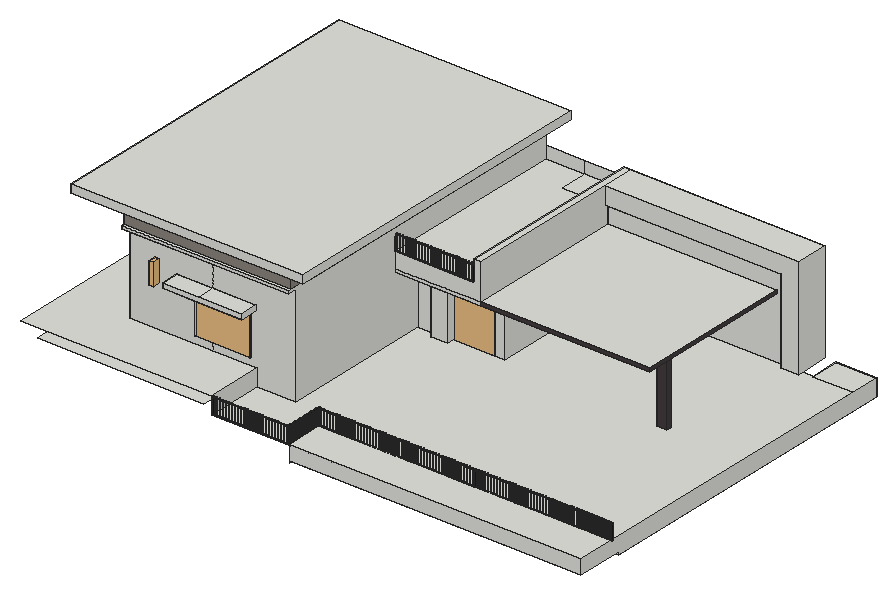
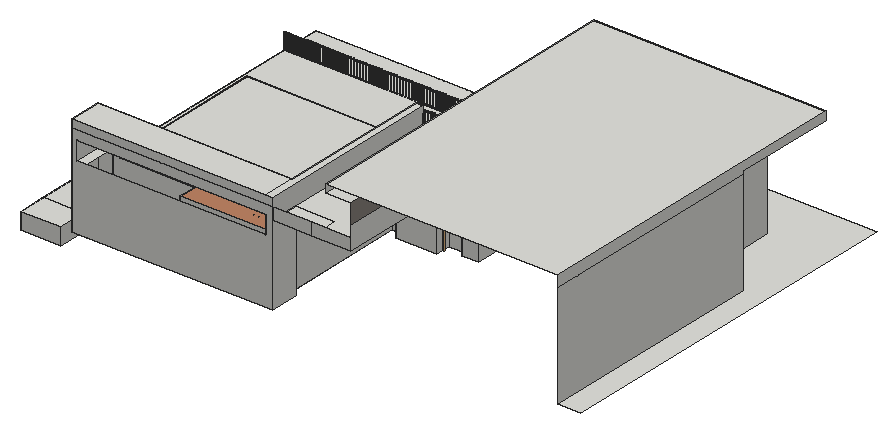
# SketchUp Ruby script. Lengths in inches.
U = 1.inch
M = Sketchup.active_model
def pt(a) = Geom::Point3d.new(a.map { |v| v * U })
def face(e, loops, mat)
  f = e.add_face(loops[0].map { |a| pt(a) })
  loops[1..].each { |l| e.add_face(l.map { |a| pt(a) }).erase! }
  f.material = f.back_material = mat if mat
  f
end
# faces: each face lists its corners as indices into pts; further lists are holes
def faces(e, pts, list, mat = nil) = list.each { |f| face(e, (f[0].is_a?(Array) ? f : [f]).map { |l| l.map { |i| pts[i] } }, mat) }
# xy, xz, yz: faces in a plane at the given z, y or x. An outline is a flat list of corners, or four numbers for a rectangle; further outlines are holes
def ring(l) = l.size == 4 ? [[l[0], l[1]], [l[2], l[1]], [l[2], l[3]], [l[0], l[3]]] : l.each_slice(2).to_a
def flat(e, list, mat, &to3) = list.each { |f| face(e, (f[0].is_a?(Array) ? f : [f]).map { |l| ring(l).map { |u, v| to3.(u, v) } }, mat) }
def xy(e, z, list, mat = nil) = flat(e, list, mat) { |x, y| [x, y, z] }
def xz(e, y, list, mat = nil) = flat(e, list, mat) { |x, z| [x, y, z] }
def yz(e, x, list, mat = nil) = flat(e, list, mat) { |y, z| [x, y, z] }
def lines(e, pts, list) = list.each { |a, b| e.add_line(pt(pts[a]), pt(pts[b])) }
# prism: a flat outline (further loops are holes) pulled along v
def prism(e, loops, v, mat = nil)
  f = face(e, loops, mat); d = Geom::Vector3d.new(v.map { |x| x * U })
  f.pushpull(f.normal.samedirection?(d) ? d.length : -d.length)
end
def box(e, o, s, mat = nil) = prism(e, [[o, [o[0] + s[0], o[1], o[2]], [o[0] + s[0], o[1] + s[1], o[2]], [o[0], o[1] + s[1], o[2]]]], [0, 0, s[2]], mat)
def at(x, y, z, deg = 0) = Geom::Transformation.translation(pt([x, y, z])) * Geom::Transformation.rotation(ORIGIN, Z_AXIS, deg.degrees)
def axes(o, x, y, z) = Geom::Transformation.new([*x, 0, *y, 0, *z, 0, *pt(o).to_a, 1])
def part(name) = M.definitions.add(name)
# library, detail: a bought-in or finely detailed component or shape, given as its bounding box
def library(name, o, s) = part(name).tap { |d| box(d.entities, o, s) }
def detail(e, o, s) = box(e.add_group.entities, o, s)
def put(e, d, t, mat = nil) = e.add_instance(d, t).tap { |i| i.material = mat if mat }
def group(e, t, mat = nil) = e.add_group.tap { |g| g.transformation = t; g.material = mat if mat }.entities
root = M.entities
M.materials.add("[Asphalt New]").color = [67, 60, 62]
M.materials.add("[Color M08]").color = [30, 30, 30]
M.materials.add("[Concrete Scored Jointless]").color = [140, 133, 127]
M.materials.add("[Modern Siding]").color = [191, 132, 100]
c1 = part("Group\#428")
prism(c1.entities,[[[0,1.97,0],[0,1.97,1.18],[0,0,1.18],[0,0,0]],[[0,1.92,1.13],[0,1.92,0.05],[0,0.05,0.05],[0,0.05,1.13]]],[98.43,0,0])
c2 = part("Group\#430")
xy(c2.entities,0,[[0.3,0,0.22,0.01,0.15,0.04,0.09,0.09,0.04,0.15,0.01,0.22,0,0.3,0.3,0.3],[0.3,0,0.3,0.3,0.59,0.3,0.58,0.22,0.55,0.15,0.5,0.09,0.44,0.04,0.37,0.01],[0,0.3,0.01,0.37,0.04,0.44,0.09,0.5,0.15,0.55,0.22,0.58,0.3,0.59,0.3,0.3],[0.3,0.3,0.3,0.59,0.37,0.58,0.44,0.55,0.5,0.5,0.55,0.44,0.58,0.37,0.59,0.3]])
xy(c2.entities,39.37,[[0.3,0,0.37,0.01,0.44,0.04,0.5,0.09,0.55,0.15,0.58,0.22,0.59,0.3,0.58,0.37,0.55,0.44,0.5,0.5,0.44,0.55,0.37,0.58,0.3,0.59,0.22,0.58,0.15,0.55,0.09,0.5,0.04,0.44,0.01,0.37,0,0.3,0.01,0.22,0.04,0.15,0.09,0.09,0.15,0.04,0.22,0.01]])
p = [[0.09,0.09,0],[0.15,0.04,0],[0.15,0.04,39.37],[0.09,0.09,39.37],[0.22,0.01,0],[0.22,0.01,39.37],
  [0.3,0,0],[0.3,0,39.37],[0.37,0.01,0],[0.37,0.01,39.37],[0.44,0.04,0],[0.44,0.04,39.37],
  [0.5,0.09,0],[0.5,0.09,39.37],[0.01,0.22,0],[0.04,0.15,0],[0.04,0.15,39.37],[0.01,0.22,39.37],
  [0.55,0.15,0],[0.55,0.15,39.37],[0.58,0.22,0],[0.58,0.22,39.37],[0,0.3,0],[0,0.3,39.37],
  [0.59,0.3,0],[0.59,0.3,39.37],[0.01,0.37,0],[0.01,0.37,39.37],[0.58,0.37,0],[0.58,0.37,39.37],
  [0.09,0.5,0],[0.04,0.44,0],[0.04,0.44,39.37],[0.09,0.5,39.37],[0.55,0.44,0],[0.5,0.5,0],
  [0.5,0.5,39.37],[0.55,0.44,39.37],[0.15,0.55,0],[0.15,0.55,39.37],[0.44,0.55,0],[0.44,0.55,39.37],
  [0.22,0.58,0],[0.22,0.58,39.37],[0.3,0.59,0],[0.3,0.59,39.37],[0.37,0.58,0],[0.37,0.58,39.37]]
faces(c2.entities,p,[[0,1,2,3],[1,4,5,2],[4,6,7,5],[6,8,9,7],[8,10,11,9],[10,12,13,11],[14,15,16,17],[15,0,3,16],
  [12,18,19,13],[18,20,21,19],[22,14,17,23],[20,24,25,21],[26,22,23,27],[24,28,29,25],[30,31,32,33],[31,26,27,32],
  [34,35,36,37],[28,34,37,29],[38,30,33,39],[35,40,41,36],[42,38,39,43],[44,42,43,45],[46,44,45,47],[40,46,47,41]])
c3 = part("Group\#429")
prism(c3.entities,[[[0.01,0.22,35.83],[0,0.3,35.83],[0.01,0.37,35.83],[0.04,0.44,35.83],[0.09,0.5,35.83],[0.15,0.55,35.83],[0.22,0.58,35.83],[0.3,0.59,35.83],[0.37,0.58,35.83],[0.44,0.55,35.83],[0.5,0.5,35.83],[0.55,0.44,35.83],[0.58,0.37,35.83],[0.59,0.3,35.83],[0.58,0.22,35.83],[0.55,0.15,35.83],[0.5,0.09,35.83],[0.44,0.04,35.83],[0.37,0.01,35.83],[0.3,0,35.83],[0.22,0.01,35.83],[0.15,0.04,35.83],[0.09,0.09,35.83],[0.04,0.15,35.83]]],[0,0,3.54])
c4 = part("Metal fence panel")
g1 = group(c4.entities,at(0,0,0))
put(g1,c1,axes([0,0,39.76],[1,0,0],[0,0,-1],[0,1,0]),"[Color M08]")
put(g1,c1,axes([0,0,1.97],[1,0,0],[0,0,-1],[0,1,0]),"[Color M08]")
put(g1,c1,axes([98.43,0,37.8],[0,0,-0.364],[-1,0,0],[0,1,0]),"[Color M08]")
put(g1,c1,axes([1.97,0,37.8],[0,0,-0.364],[-1,0,0],[0,1,0]),"[Color M08]")
g2 = group(c4.entities,at(1.67,0.3,1.97))
put(g2,c2,at(78.74,0,0),"[Color M08]")
put(g2,c2,at(90.55,0,0),"[Color M08]")
put(g2,c2,at(82.68,0,0),"[Color M08]")
put(g2,c2,at(86.61,0,0),"[Color M08]")
put(g2,c2,at(66.93,0,0),"[Color M08]")
put(g2,c2,at(11.8125,0,0),"[Color M08]")
put(g2,c2,at(15.75,0,0),"[Color M08]")
put(g2,c2,at(47.24,0,0),"[Color M08]")
put(g2,c2,at(59.06,0,0),"[Color M08]")
put(g2,c3,at(0,0,0),"[Color M08]")
put(g2,c2,at(39.37,0,0),"[Color M08]")
put(g2,c2,at(62.99,0,0),"[Color M08]")
put(g2,c2,at(55.12,0,0),"[Color M08]")
put(g2,c2,at(19.69,0,0),"[Color M08]")
put(g2,c2,at(35.43,0,0),"[Color M08]")
put(g2,c2,at(7.875,0,0),"[Color M08]")
put(g2,c2,at(23.62,0,0),"[Color M08]")
put(g2,c2,at(31.5,0,0),"[Color M08]")
put(g2,c2,at(43.31,0,0),"[Color M08]")
put(g2,c2,at(27.56,0,0),"[Color M08]")
put(g2,c2,at(3.9375,0,0),"[Color M08]")
put(g2,c2,at(51.18,0,0),"[Color M08]")
put(g2,c2,at(70.87,0,0),"[Color M08]")
put(g2,c2,at(74.8,0,0),"[Color M08]")
put(g2,c3,at(94.49,0,0),"[Color M08]")
c5 = library("window\#2",[0,0,0],[78.15,10.2,70.87])
c6 = part("Senza")
g3 = group(c6.entities,at(-137.05,828.91,-82.14))
detail(g3,[0,0,0],[37.72,1.46,81.14])
c7 = library("Thorburn+Narrow+Wall+Sconce+-+Dark+Aluminum",[0,-1.5,-7.55],[4.87,3,15.1])
xy(root,225.29,[[971.9,521.59,971.9,572.2,983.57,572.2,983.66,571.52,983.93,570.89,984.34,570.35,984.89,569.93,985.52,569.67,986.2,569.58,986.88,569.67,987.51,569.93,988.06,570.35,988.47,570.89,988.73,571.52,988.82,572.2,1028.51,572.2,1028.6,571.52,1028.86,570.89,1029.28,570.35,1029.82,569.93,1030.46,569.67,1031.14,569.58,1031.82,569.67,1032.45,569.93,1032.99,570.35,1033.41,570.89,1033.67,571.52,1033.76,572.2,1073.45,572.2,1073.54,571.52,1073.8,570.89,1074.22,570.35,1074.76,569.93,1075.39,569.67,1076.07,569.58,1076.75,569.67,1077.39,569.93,1077.93,570.35,1078.35,570.89,1078.61,571.52,1078.7,572.2,1118.39,572.2,1118.48,571.52,1118.74,570.89,1119.16,570.35,1119.7,569.93,1120.33,569.67,1121.01,569.58,1121.69,569.67,1122.32,569.93,1122.87,570.35,1123.28,570.89,1123.55,571.52,1123.64,572.2,1163.32,572.2,1163.41,571.52,1163.68,570.89,1164.09,570.35,1164.64,569.93,1165.27,569.67,1165.95,569.58,1166.63,569.67,1167.26,569.93,1167.81,570.35,1168.22,570.89,1168.48,571.52,1168.57,572.2,1208.26,572.2,1208.35,571.52,1208.61,570.89,1209.03,570.35,1209.57,569.93,1210.21,569.67,1210.89,569.58,1211.57,569.67,1212.2,569.93,1212.74,570.35,1213.16,570.89,1213.42,571.52,1213.51,572.2,1253.2,572.2,1253.29,571.52,1253.55,570.89,1253.97,570.35,1254.51,569.93,1255.14,569.67,1255.82,569.58,1256.5,569.67,1257.14,569.93,1257.68,570.35,1258.1,570.89,1258.36,571.52,1258.45,572.2,1298.14,572.2,1298.23,571.52,1298.49,570.89,1298.91,570.35,1299.45,569.93,1300.08,569.67,1300.76,569.58,1301.44,569.67,1302.07,569.93,1302.62,570.35,1303.03,570.89,1303.3,571.52,1303.39,572.2,1343.07,572.2,1343.16,571.52,1343.43,570.89,1343.84,570.35,1344.39,569.93,1345.02,569.67,1345.7,569.58,1346.38,569.67,1347.01,569.93,1347.56,570.35,1347.97,570.89,1348.23,571.52,1348.32,572.2,1388.01,572.2,1388.1,571.52,1388.36,570.89,1388.78,570.35,1389.32,569.93,1389.96,569.67,1390.64,569.58,1391.32,569.67,1391.95,569.93,1392.49,570.35,1392.91,570.89,1393.17,571.52,1393.26,572.2,1425.51,572.2,1425.51,521.59],[1443.95,521.59,1520.01,1128.33],[986.2,569.58,985.52,569.67,984.89,569.93,984.34,570.35,983.93,570.89,983.66,571.52,983.57,572.2,988.82,572.2,988.73,571.52,988.47,570.89,988.06,570.35,987.51,569.93,986.88,569.67],[1031.14,569.58,1030.46,569.67,1029.82,569.93,1029.28,570.35,1028.86,570.89,1028.6,571.52,1028.51,572.2,1033.76,572.2,1033.67,571.52,1033.41,570.89,1032.99,570.35,1032.45,569.93,1031.82,569.67],[1076.07,569.58,1075.39,569.67,1074.76,569.93,1074.22,570.35,1073.8,570.89,1073.54,571.52,1073.45,572.2,1078.7,572.2,1078.61,571.52,1078.35,570.89,1077.93,570.35,1077.39,569.93,1076.75,569.67],
  [1121.01,569.58,1120.33,569.67,1119.7,569.93,1119.16,570.35,1118.74,570.89,1118.48,571.52,1118.39,572.2,1123.64,572.2,1123.55,571.52,1123.28,570.89,1122.87,570.35,1122.32,569.93,1121.69,569.67],[1165.95,569.58,1165.27,569.67,1164.64,569.93,1164.09,570.35,1163.68,570.89,1163.41,571.52,1163.32,572.2,1168.57,572.2,1168.48,571.52,1168.22,570.89,1167.81,570.35,1167.26,569.93,1166.63,569.67],[1210.89,569.58,1210.21,569.67,1209.57,569.93,1209.03,570.35,1208.61,570.89,1208.35,571.52,1208.26,572.2,1213.51,572.2,1213.42,571.52,1213.16,570.89,1212.74,570.35,1212.2,569.93,1211.57,569.67],[1255.82,569.58,1255.14,569.67,1254.51,569.93,1253.97,570.35,1253.55,570.89,1253.29,571.52,1253.2,572.2,1258.45,572.2,1258.36,571.52,1258.1,570.89,1257.68,570.35,1257.14,569.93,1256.5,569.67],[1300.76,569.58,1300.08,569.67,1299.45,569.93,1298.91,570.35,1298.49,570.89,1298.23,571.52,1298.14,572.2,1303.39,572.2,1303.3,571.52,1303.03,570.89,1302.62,570.35,1302.07,569.93,1301.44,569.67],
  [1345.7,569.58,1345.02,569.67,1344.39,569.93,1343.84,570.35,1343.43,570.89,1343.16,571.52,1343.07,572.2,1348.32,572.2,1348.23,571.52,1347.97,570.89,1347.56,570.35,1347.01,569.93,1346.38,569.67],[971.9,572.2,971.9,719.78,1074.08,714.35,1176.26,714.35,1176.26,719.78,1332.64,719.78,1332.64,714.35,1425.51,714.35,1425.51,572.2,1393.26,572.2,1393.17,572.88,1392.91,573.52,1392.49,574.06,1391.95,574.48,1391.32,574.74,1390.64,574.83,1389.96,574.74,1389.32,574.48,1388.78,574.06,1388.36,573.52,1388.1,572.88,1388.01,572.2,1348.32,572.2,1348.23,572.88,1347.97,573.52,1347.56,574.06,1347.01,574.48,1346.38,574.74,1345.7,574.83,1345.02,574.74,1344.39,574.48,1343.84,574.06,1343.43,573.52,1343.16,572.88,1343.07,572.2,1303.39,572.2,1303.3,572.88,1303.03,573.52,1302.62,574.06,1302.07,574.48,1301.44,574.74,1300.76,574.83,1300.08,574.74,1299.45,574.48,1298.91,574.06,1298.49,573.52,1298.23,572.88,1298.14,572.2,1258.45,572.2,1258.36,572.88,1258.1,573.52,1257.68,574.06,1257.14,574.48,1256.5,574.74,1255.82,574.83,1255.14,574.74,1254.51,574.48,1253.97,574.06,1253.55,573.52,1253.29,572.88,1253.2,572.2,1213.51,572.2,1213.42,572.88,1213.16,573.52,1212.74,574.06,1212.2,574.48,1211.57,574.74,1210.89,574.83,1210.21,574.74,1209.57,574.48,1209.03,574.06,1208.61,573.52,1208.35,572.88,1208.26,572.2,1168.57,572.2,1168.48,572.88,1168.22,573.52,1167.81,574.06,1167.26,574.48,1166.63,574.74,1165.95,574.83,1165.27,574.74,1164.64,574.48,1164.09,574.06,1163.68,573.52,1163.41,572.88,1163.32,572.2,1123.64,572.2,1123.55,572.88,1123.28,573.52,1122.87,574.06,1122.32,574.48,1121.69,574.74,1121.01,574.83,1120.33,574.74,1119.7,574.48,1119.16,574.06,1118.74,573.52,1118.48,572.88,1118.39,572.2,1078.7,572.2,1078.61,572.88,1078.35,573.52,1077.93,574.06,1077.39,574.48,1076.75,574.74,1076.07,574.83,1075.39,574.74,1074.76,574.48,1074.22,574.06,1073.8,573.52,1073.54,572.88,1073.45,572.2,1033.76,572.2,1033.67,572.88,1033.41,573.52,1032.99,574.06,1032.45,574.48,1031.82,574.74,1031.14,574.83,1030.46,574.74,1029.82,574.48,1029.28,574.06,1028.86,573.52,1028.6,572.88,1028.51,572.2,988.82,572.2,988.73,572.88,988.47,573.52,988.06,574.06,987.51,574.48,986.88,574.74,986.2,574.83,985.52,574.74,984.89,574.48,984.34,574.06,983.93,573.52,983.66,572.88,983.57,572.2],[983.57,572.2,983.66,572.88,983.93,573.52,984.34,574.06,984.89,574.48,985.52,574.74,986.2,574.83,986.88,574.74,987.51,574.48,988.06,574.06,988.47,573.52,988.73,572.88,988.82,572.2],[1028.51,572.2,1028.6,572.88,1028.86,573.52,1029.28,574.06,1029.82,574.48,1030.46,574.74,1031.14,574.83,1031.82,574.74,1032.45,574.48,1032.99,574.06,1033.41,573.52,1033.67,572.88,1033.76,572.2],[1073.45,572.2,1073.54,572.88,1073.8,573.52,1074.22,574.06,1074.76,574.48,1075.39,574.74,1076.07,574.83,1076.75,574.74,1077.39,574.48,1077.93,574.06,1078.35,573.52,1078.61,572.88,1078.7,572.2],
  [1118.39,572.2,1118.48,572.88,1118.74,573.52,1119.16,574.06,1119.7,574.48,1120.33,574.74,1121.01,574.83,1121.69,574.74,1122.32,574.48,1122.87,574.06,1123.28,573.52,1123.55,572.88,1123.64,572.2],[1163.32,572.2,1163.41,572.88,1163.68,573.52,1164.09,574.06,1164.64,574.48,1165.27,574.74,1165.95,574.83,1166.63,574.74,1167.26,574.48,1167.81,574.06,1168.22,573.52,1168.48,572.88,1168.57,572.2],[1208.26,572.2,1208.35,572.88,1208.61,573.52,1209.03,574.06,1209.57,574.48,1210.21,574.74,1210.89,574.83,1211.57,574.74,1212.2,574.48,1212.74,574.06,1213.16,573.52,1213.42,572.88,1213.51,572.2],[1253.2,572.2,1253.29,572.88,1253.55,573.52,1253.97,574.06,1254.51,574.48,1255.14,574.74,1255.82,574.83,1256.5,574.74,1257.14,574.48,1257.68,574.06,1258.1,573.52,1258.36,572.88,1258.45,572.2],[1298.14,572.2,1298.23,572.88,1298.49,573.52,1298.91,574.06,1299.45,574.48,1300.08,574.74,1300.76,574.83,1301.44,574.74,1302.07,574.48,1302.62,574.06,1303.03,573.52,1303.3,572.88,1303.39,572.2],
  [1343.07,572.2,1343.16,572.88,1343.43,573.52,1343.84,574.06,1344.39,574.48,1345.02,574.74,1345.7,574.83,1346.38,574.74,1347.01,574.48,1347.56,574.06,1347.97,573.52,1348.23,572.88,1348.32,572.2],[1074.08,714.35,971.9,719.78,1074.08,719.78]])
xy(root,230.06,[[971.9,433.09,1520.01,521.59]])
xy(root,256.3125,[[[825.44,433.09,1520.01,433.09,1520.01,1073.99,1423.77,1073.99,1423.77,1065.37,1390.19,1065.37,1390.19,1073.99,1058.71,1073.99,1058.71,830.55,1040.11,830.55,1040.11,845.87,963.03,845.87,963.03,817.18,930.75,817.18,930.75,826.49,898.67,826.49,898.67,540.08,825.44,540.08],[1358.52,813.98,1377.07,824.35]],[1045.74,1073.99,1045.74,1128.33,1423.77,1128.33,1423.77,1073.99,1235.8,1073.99,1235.8,1107.24,1058.71,1107.24,1058.71,1073.99],[1058.71,1073.99,1235.8,1107.24],[1443.95,1073.99,1520.01,1128.33]])
xy(root,269.5625,[[497.32,433.09,810.8,490.53]])
xy(root,287.9375,[[465.27,433.09,825.44,433.09,825.44,540.08,584.86,540.08,584.86,693.95,507.79,693.95,507.79,1128.33,465.27,1128.33]])
xy(root,300.07,[[708.1,540.08,741.76,615.96],[741.76,540.08,812.1,615.96]])
xy(root,372.6875,[[1358.52,773.43,1377.07,813.98],[1358.52,813.98,1377.07,824.35]])
xy(root,372.6875,[[898.67,773.43,930.75,826.49],[930.75,773.43,963.03,817.18],[963.03,773.43,1040.11,845.87],[1040.11,773.43,1058.71,830.55],[1058.71,773.43,1058.71,1107.24,1235.8,1107.24,1235.8,1073.99,1377.07,1073.99,1377.07,824.35,1358.52,824.35,1358.52,773.43]],"[Modern Siding]")
xy(root,378.5,[[1058.71,773.43,1377.07,1073.99],[1397.33,1073.99,1413.6,1128.33]])
xy(root,383.2,[[674.45,507.46,741.76,540.08],[741.76,507.46,823.38,540.08],[708.1,540.08,741.76,615.96],[741.76,540.08,812.1,615.96]])
xy(root,393.26,[[674.45,507.46,741.76,540.08],[741.76,507.46,823.38,540.08]])
xy(root,407.9375,[[898.67,773.43,1045.74,773.43,1045.74,1073.99,971.9,1073.99,971.9,1128.33,898.67,1128.33],[971.9,1073.99,1045.74,1128.33]])
xy(root,414.625,[[1058.71,1065.37,1058.71,1073.99,1390.19,1073.99,1390.19,1073.43,1377.07,1073.43,1377.07,1065.37],[1377.07,1065.37,1390.19,1073.43],[1058.71,1073.99,1413.6,1128.33]])
xy(root,445.75,[[1045.74,773.43,1058.71,1128.33],[1058.71,1065.37,1423.77,1128.33]])
xy(root,446.51,[[584.86,521.96,898.67,540.08]])
xy(root,451.4375,[[584.86,521.96,898.67,527.6875]])
xy(root,488.97,[[507.79,499.14,944.67,527.6875],[507.79,527.6875,584.86,693.95],[898.67,527.6875,944.67,1128.33]])
xy(root,504.5,[[507.79,499.14,944.67,1128.33]])
xz(root,433.09,[[971.9,230.06,1520.01,256.3125]])
xz(root,499.14,[[507.79,488.97,944.67,504.5]])
xz(root,507.46,[[674.45,383.2,823.38,393.26]])
xz(root,521.59,[[971.9,225.29,1520.01,230.06]])
xz(root,521.96,[[584.86,446.51,898.67,451.4375]])
xz(root,527.6875,[[584.86,451.4375,898.67,488.97]],"[Concrete Scored Jointless]")
xz(root,540.08,[[825.44,256.3125,898.67,256.3125,898.67,446.51,741.76,446.51,741.76,393.26,823.38,393.26,823.38,383.2,812.1,383.2,812.1,300.07,741.76,300.07,741.76,287.9375,825.44,287.9375],[584.86,287.9375,741.76,287.9375,741.76,300.07,708.1,300.07,708.1,383.2,674.45,383.2,674.45,393.26,741.76,393.26,741.76,446.51,584.86,446.51],[674.45,383.2,823.38,393.26]])
xz(root,615.96,[[708.1,300.07,812.1,383.2]])
xz(root,693.95,[[507.79,287.9375,584.86,488.97]])
xz(root,773.43,[[898.67,372.6875,1058.71,378.5],[898.67,378.5,1058.71,378.5,1058.71,445.75,1045.74,445.75,1045.74,407.9375,898.67,407.9375]])
xz(root,773.43,[[1058.71,372.6875,1377.07,378.5]],"[Asphalt New]")
xz(root,813.98,[[1358.52,256.3125,1377.07,372.6875]],"[Asphalt New]")
xz(root,817.18,[[930.75,256.3125,963.03,372.6875]])
xz(root,824.35,[[1358.52,256.3125,1377.07,372.6875]],"[Asphalt New]")
xz(root,826.49,[[898.67,256.3125,930.75,372.6875]])
xz(root,830.55,[[1040.11,256.3125,1058.71,372.6875]])
xz(root,845.87,[[963.03,256.3125,1040.11,372.6875]])
xz(root,1065.37,[[1390.19,256.3125,1423.77,256.3125,1423.77,445.75,1058.71,445.75,1058.71,414.625,1390.19,414.625]])
xz(root,1073.99,[[1235.8,256.3125,1235.8,372.6875,1377.07,372.6875,1377.07,378.5,1058.71,378.5,1058.71,414.625,1390.19,414.625,1390.19,256.3125],[1390.19,378.5,1413.6,414.625]])
xz(root,1107.24,[[1058.71,256.3125,1235.8,372.6875]])
xz(root,1128.33,[[1443.95,225.29,1520.01,256.3125],[[1045.74,256.3125,1423.77,430.5],[1058.71,378.5,1413.6,414.625]],[898.67,407.9375,971.9,430.5],[971.9,407.9375,1045.74,430.5],[1045.74,430.5,1423.77,445.75]])
yz(root,507.79,[[693.95,287.9375,1128.33,482.59],[693.95,482.59,693.95,488.97,499.14,488.97,499.14,504.5,1128.33,504.5,1128.33,482.59]])
yz(root,584.86,[[540.08,287.9375,540.08,446.51,521.96,446.51,521.96,451.4375,693.95,451.4375,693.95,287.9375]])
yz(root,584.86,[[527.6875,451.4375,693.95,488.97]],"[Concrete Scored Jointless]")
yz(root,674.45,[[507.46,383.2,540.08,393.26]])
yz(root,708.1,[[540.08,300.07,615.96,383.2]])
yz(root,812.1,[[540.08,300.07,615.96,383.2]])
yz(root,823.38,[[507.46,383.2,540.08,393.26]])
yz(root,825.44,[[433.09,256.3125,540.08,287.9375]])
yz(root,898.67,[[540.08,256.3125,826.49,256.3125,826.49,372.6875,773.43,372.6875,773.43,407.9375,1128.33,407.9375,1128.33,451.4375,521.96,451.4375,521.96,446.51,540.08,446.51]])
yz(root,898.67,[[527.6875,451.4375,1128.33,488.97]],"[Concrete Scored Jointless]")
yz(root,930.75,[[817.18,256.3125,826.49,372.6875]])
yz(root,944.67,[[499.14,488.97,1128.33,504.5]])
yz(root,963.03,[[817.18,256.3125,845.87,372.6875]])
yz(root,971.9,[[433.09,225.29,521.59,230.06]])
yz(root,1040.11,[[830.55,256.3125,845.87,372.6875]])
yz(root,1045.74,[[1073.99,256.3125,1128.33,407.9375],[773.43,407.9375,1128.33,445.75]])
yz(root,1058.71,[[830.55,256.3125,1107.24,372.6875],[773.43,378.5,1073.99,378.5,1073.99,414.625,1065.37,414.625,1065.37,445.75,773.43,445.75],[1073.99,378.5,1128.33,414.625]])
yz(root,1235.8,[[1073.99,256.3125,1107.24,372.6875]])
yz(root,1358.52,[[813.98,256.3125,824.35,372.6875]],"[Asphalt New]")
yz(root,1377.07,[[813.98,256.3125,824.35,372.6875],[773.43,372.6875,1073.99,378.5]],"[Asphalt New]")
yz(root,1390.19,[[1065.37,256.3125,1073.99,378.5],[1065.37,378.5,1073.43,414.625],[1073.43,378.5,1073.99,414.625]])
yz(root,1413.6,[[1073.99,378.5,1128.33,414.625]])
yz(root,1423.77,[[1065.37,256.3125,1128.33,445.75]])
yz(root,1443.95,[[1073.99,225.29,1128.33,256.3125]])
yz(root,1520.01,[[521.59,225.29,1128.33,225.29,1128.33,256.3125,433.09,256.3125,433.09,230.06,521.59,230.06]])
p = [[971.9,567.36,205.26],[971.9,567.1,204.64],[1428.71,567.1,204.64],[1428.71,567.36,205.26],[971.9,572.05,204.64],[971.9,571.8,205.26],
  [1428.71,571.8,205.26],[1428.71,572.05,204.64],[971.9,567.77,205.79],[1428.71,567.77,205.79],[971.9,571.39,205.79],[1428.71,571.39,205.79],
  [971.9,568.3,206.2],[1428.71,568.3,206.2],[971.9,570.86,206.2],[1428.71,570.86,206.2],[971.9,568.92,206.46],[1428.71,568.92,206.46],
  [971.9,570.24,206.46],[1428.71,570.24,206.46],[971.9,569.58,206.54],[1428.71,569.58,206.54],[1390.64,569.58,206.54],[1345.7,569.58,206.54],
  [1300.76,569.58,206.54],[1255.82,569.58,206.54],[1210.89,569.58,206.54],[1165.95,569.58,206.54],[1121.01,569.58,206.54],[1076.07,569.58,206.54],
  [1031.14,569.58,206.54],[986.2,569.58,206.54],[1423.77,1128.33,364.125],[1413.6,1128.33,364.125],[1413.6,1073.99,364.125],[938.64,572.2,225.29],
  [943.89,572.2,225.29],[1390.19,1073.43,372.6875],[1390.19,1073.99,372.6875]]
faces(root,p,[[0,1,2,3],[4,5,6,7],[8,0,3,9],[5,10,11,6],[12,8,9,13],[10,14,15,11],[16,12,13,17],[14,18,19,15],
  [20,16,17,21,22,23,24,25,26,27,28,29,30,31],[18,20,31,30,29,28,27,26,25,24,23,22,21,19]])
lines(root,p,[[32,33],[34,33],[35,36],[37,38]])
put(root,c4,axes([1405.15,505.6,254.8],[1.17433,0,0],[0,0.77,0],[0,0,0.77]))
put(root,c4,axes([969.46,505.6,254.8],[1.46791,0,0],[0,0.77,0],[0,0,0.77]))
put(root,c4,axes([1116.84,505.6,254.8],[1.46791,0,0],[0,0.77,0],[0,0,0.77]))
put(root,c4,axes([1260.27,505.6,254.8],[1.46791,0,0],[0,0.77,0],[0,0,0.77]))
put(root,c5,axes([1058.71,1070.85,254.87],[2.266,0,0],[0,1.188,0],[0,0,1.64916]))
put(root,c6,axes([1252.14,-444.73,404.99],[2.13447,0,0],[0,1.5385,0],[0,0,1.81]))
put(root,c4,axes([825.44,433.09,256.3125],[1.46791,0,0],[0,0.77,0],[0,0,0.77]))
put(root,c4,axes([969.92,433.09,256.3125],[0,0.74908,0],[-0.77,0,0],[0,0,0.77]))
put(root,c5,axes([708.1,541.3,300.07],[1.34042,0,0],[0,0.88,0],[0,0,1.2216]))
put(root,c7,axes([636.91,540.06,386.35],[0,-2.73,0],[2.73,0,0],[0,0,2.73]))
put(root,c4,axes([898.67,773.43,407.9375],[1.49427,0,0],[0,-0.42319,0],[0,0,0.77]))
